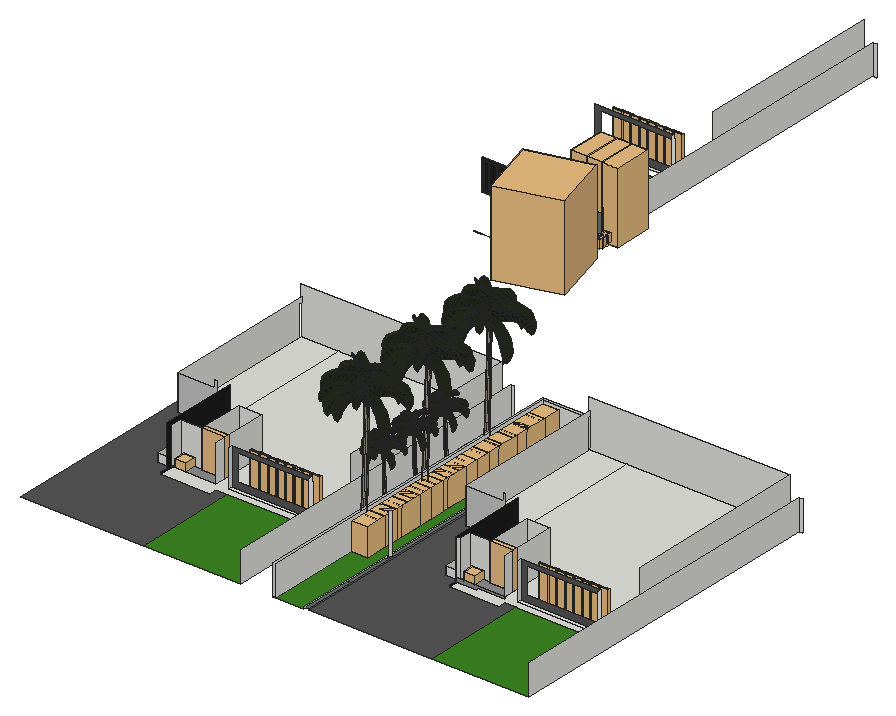
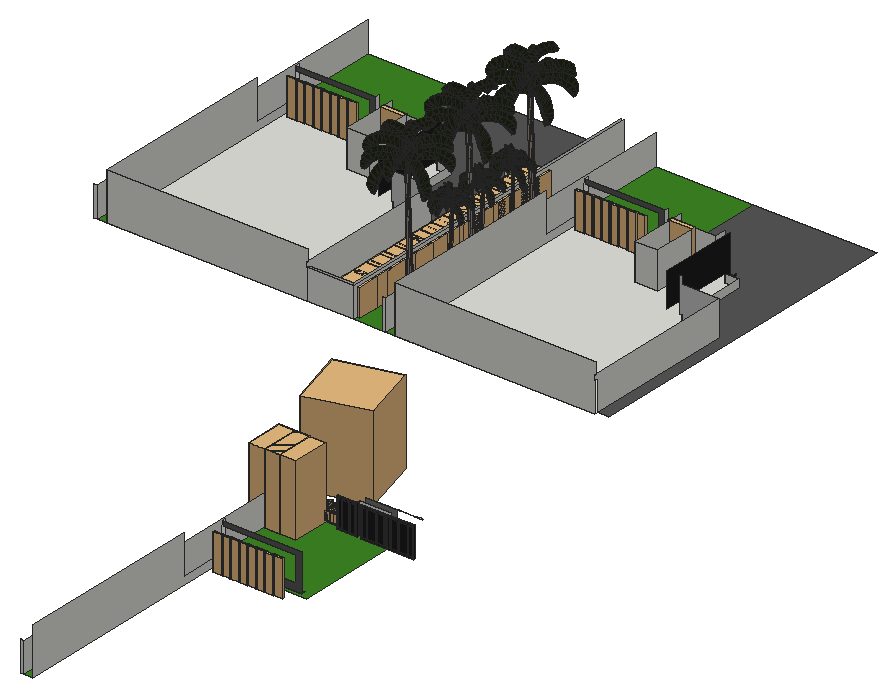
# SketchUp Ruby script. Lengths in inches.
U = 1.inch
M = Sketchup.active_model
def pt(a) = Geom::Point3d.new(a.map { |v| v * U })
def face(e, loops, mat)
  f = e.add_face(loops[0].map { |a| pt(a) })
  loops[1..].each { |l| e.add_face(l.map { |a| pt(a) }).erase! }
  f.material = f.back_material = mat if mat
  f
end
# faces: each face lists its corners as indices into pts; further lists are holes
def faces(e, pts, list, mat = nil) = list.each { |f| face(e, (f[0].is_a?(Array) ? f : [f]).map { |l| l.map { |i| pts[i] } }, mat) }
# xy, xz, yz: faces in a plane at the given z, y or x. An outline is a flat list of corners, or four numbers for a rectangle; further outlines are holes
def ring(l) = l.size == 4 ? [[l[0], l[1]], [l[2], l[1]], [l[2], l[3]], [l[0], l[3]]] : l.each_slice(2).to_a
def flat(e, list, mat, &to3) = list.each { |f| face(e, (f[0].is_a?(Array) ? f : [f]).map { |l| ring(l).map { |u, v| to3.(u, v) } }, mat) }
def xy(e, z, list, mat = nil) = flat(e, list, mat) { |x, y| [x, y, z] }
def xz(e, y, list, mat = nil) = flat(e, list, mat) { |x, z| [x, y, z] }
def yz(e, x, list, mat = nil) = flat(e, list, mat) { |y, z| [x, y, z] }
def lines(e, pts, list) = list.each { |a, b| e.add_line(pt(pts[a]), pt(pts[b])) }
# prism: a flat outline (further loops are holes) pulled along v
def prism(e, loops, v, mat = nil)
  f = face(e, loops, mat); d = Geom::Vector3d.new(v.map { |x| x * U })
  f.pushpull(f.normal.samedirection?(d) ? d.length : -d.length)
end
def box(e, o, s, mat = nil) = prism(e, [[o, [o[0] + s[0], o[1], o[2]], [o[0] + s[0], o[1] + s[1], o[2]], [o[0], o[1] + s[1], o[2]]]], [0, 0, s[2]], mat)
def at(x, y, z, deg = 0) = Geom::Transformation.translation(pt([x, y, z])) * Geom::Transformation.rotation(ORIGIN, Z_AXIS, deg.degrees)
def axes(o, x, y, z) = Geom::Transformation.new([*x, 0, *y, 0, *z, 0, *pt(o).to_a, 1])
def part(name) = M.definitions.add(name)
# library, detail: a bought-in or finely detailed component or shape, given as its bounding box
def library(name, o, s) = part(name).tap { |d| box(d.entities, o, s) }
def detail(e, o, s) = box(e.add_group.entities, o, s)
def put(e, d, t, mat = nil) = e.add_instance(d, t).tap { |i| i.material = mat if mat }
def group(e, t, mat = nil) = e.add_group.tap { |g| g.transformation = t; g.material = mat if mat }.entities
root = M.entities
M.materials.add("Antracyt").color = [44, 47, 50]
M.materials.add("Carpet_Ltblue").color = [157, 173, 165]
M.materials.add("Manila2").color = [36, 43, 22]
M.materials.add("ManilaTruck").color = [158, 143, 128]
M.materials.add("[Color M00]").color = [255, 255, 255]
M.materials.add("[Color M02]").color = [198, 198, 198]
M.materials.add("[Color M04]").color = [60, 133, 34]
M.materials.add("[Color M04]1").color = [142, 142, 142]
M.materials.add("[Color M05]1").color = [114, 114, 114]
M.materials.add("[Color M06]1").color = [86, 86, 86]
M.materials.add("[Color M08]").color = [30, 30, 30]
M.materials.add("[Color_F16]").color = [51, 102, 0]
M.materials.add("[Field Square Tile]").color = [217, 201, 169]
M.materials.add("[Slate Light Tile]").color = [86, 86, 86]
M.materials.add("[Slate]").color = [102, 110, 108]
c1 = part("Group\#102")
g1 = group(c1.entities,at(0,0,0))
prism(g1,[[[0,3,72],[70.5,3,72],[70.5,3,0],[0,3,0]],[[67.5,3,3],[67.5,3,69],[3,3,69],[3,3,3]]],[0,-3,0])
c2 = part("Group\#135")
box(c2.entities,[0,0,0],[0.5,1,66])
c3 = part("Group\#148")
box(c3.entities,[0,-1,0],[5.5,1,66])
box(c3.entities,[50.84,-1,0],[13.66,1,66])
box(c3.entities,[28.06,-1,0],[22.28,1,66])
box(c3.entities,[24.66,-1,0],[2.9,1,66])
box(c3.entities,[6,-1,0],[18.16,1,66])
c4 = part("Component\#23")
g2 = group(c4.entities,at(70.5,0,0),"[Color M08]")
put(g2,c1,axes([70.5,0,0],[-1,0,0],[0,1,0],[0,0,1]))
g3 = group(g2,at(3,2,3))
g4 = group(g3,at(0,-1,0))
box(g4,[0,0,0],[5.5,1,66])
box(g4,[50.84,0,0],[13.66,1,66])
box(g4,[28.06,0,0],[22.28,1,66])
box(g4,[24.66,0,0],[2.9,1,66])
box(g4,[6,0,0],[18.16,1,66])
put(g3,c2,axes([50.34,0,0],[1,0,0],[0,-1,0],[0,0,1]))
put(g3,c2,axes([24.16,0,0],[1,0,0],[0,-1,0],[0,0,1]))
put(g3,c2,axes([27.56,0,0],[1,0,0],[0,-1,0],[0,0,1]))
put(g3,c2,axes([5.5,0,0],[1,0,0],[0,-1,0],[0,0,1]))
g5 = group(c4.entities,at(70.5,0,0),"[Color M08]")
put(g5,c1,at(-70.5,0,0))
g6 = group(g5,at(-3,2,3,-180))
put(g6,c3,at(0,1,0))
put(g6,c2,at(50.34,0,0))
put(g6,c2,at(24.16,0,0))
put(g6,c2,at(27.56,0,0))
put(g6,c2,at(5.5,0,0))
g7 = group(c4.entities,at(150,0,0),"[Color M08]")
put(g7,c1,axes([54,0,0],[-0.76596,0,0],[0,1,0],[0,0,1]))
g8 = group(g7,at(2.3,2,3))
put(g8,c3,axes([0,-1,0],[0.76596,0,0],[0,-1,0],[0,0,1]))
put(g8,c2,axes([38.55,0,0],[0.76596,0,0],[0,-1,0],[0,0,1]))
put(g8,c2,axes([18.5,0,0],[0.76596,0,0],[0,-1,0],[0,0,1]))
put(g8,c2,axes([21.11,0,0],[0.76596,0,0],[0,-1,0],[0,0,1]))
put(g8,c2,axes([4.22,0,0],[0.76596,0,0],[0,-1,0],[0,0,1]))
c5 = library("Group\#1",[0,0,0],[29.75,5.78,110.95])
c6 = library("Obj_000004",[-25.54,-25.36,-14.31],[50.67,50.64,41.42])
c7 = library("Obj_000003",[-31,-31.06,-7.89],[62,62.12,39.58])
c8 = library("建立群組\#17",[-3.75,-3.74,-0.43],[25.39,25.39,17.69])
c9 = library("Potted plant",[-29.7,0,-10.87],[31.67,38.52,72.45])
c10 = library("Palm tree",[-4.09,-4.52,0],[193.52,193.51,258.93])
c11 = part("Palm+Tree")
put(c11.entities,c10,at(25.51,-21.81,0,15))
c12 = library("modern+door",[0,0,0],[59.06,11.8125,86.61])
c13 = part("P_trunck")
xz(c13.entities,2.71,[[7.39,73.15,8.49,73.15,9.26,91.63,8.16,91.63]],"ManilaTruck")
xz(c13.entities,6.09,[[3.91,10.2,7.39,73.15,8.49,73.15,5.33,10.2],[7.39,73.15,8.16,91.63,9.26,91.63,8.49,73.15]],"ManilaTruck")
p = [[3.19,0,0],[3.91,1.7,10.2],[2.75,2.54,10.2],[0.88,1.68,0],[6.05,0,0],[5.33,1.7,10.2],
  [8.36,1.68,0],[6.49,2.54,10.2],[2.31,3.9,10.2],[0,4.39,0],[9.24,4.39,0],[6.93,3.9,10.2],
  [2.75,5.25,10.2],[0.88,7.11,0],[8.36,7.11,0],[6.49,5.25,10.2],[3.91,6.09,10.2],[3.19,8.79,0],
  [6.05,8.79,0],[5.33,6.09,10.2],[7.39,2.71,73.15],[6.5,3.36,73.15],[8.49,2.71,73.15],[9.38,3.36,73.15],
  [6.16,4.4,73.15],[9.72,4.4,73.15],[6.5,5.45,73.15],[9.38,5.45,73.15],[7.39,6.09,73.15],[8.49,6.09,73.15],
  [8.16,2.71,91.63],[7.27,3.36,91.63],[10.15,3.36,91.63],[9.26,2.71,91.63],[6.93,4.4,91.63],[10.49,4.4,91.63],
  [7.27,5.45,91.63],[10.15,5.45,91.63],[8.16,6.09,91.63],[9.26,6.09,91.63]]
faces(c13.entities,p,[[0,1,2,3],[4,5,1,0],[6,7,5,4],[3,2,8,9],[6,10,11,7],[8,12,13,9],[11,10,14,15],[13,12,16,17],
  [18,19,15,14],[17,16,19,18],[1,20,21,2],[5,22,20,1],[7,23,22,5],[2,21,24,8],[7,11,25,23],[8,24,26,12],
  [11,15,27,25],[12,26,28,16],[19,29,27,15],[20,30,31,21],[23,32,33,22],[31,34,24,21],[23,25,35,32],[34,36,26,24],
  [25,27,37,35],[26,36,38,28],[29,39,37,27]],"ManilaTruck")
c14 = part("halfleave")
p = [[3.15,0,0],[0.57,2.5,1.86],[4.875,1.71,0],[46.16,1.62,0],[42.0625,6.98,0],[45.79,16.25,3.85],
  [48.16,12.12,1.98],[48.16,1.62,0],[6.6,3.42,0],[-0.25,5.68,3.48],[9.02,6.6,0],[-0.31,11.68,4.96],
  [2.05,16.625,5.9],[10.99,8.52,0],[36.71,10.67,0],[41.5,21.18,5.01],[8.2,21.17,6.52],[12.96,10.44,0],
  [15.16,24.88,6.8125],[17.61,12.89,0],[31.19,13.02,0],[36.16,23.66,5.26],[19.91,24.88,6.5625],[20.53,13.55,0],
  [25.77,13.9375,0],[30.57,24.88,6.0625],[25.21,24.88,6.26]]
faces(c14.entities,p,[[0,1,2],[3,4,5],[5,6,3],[7,3,6],[2,1,8],[9,8,1],[8,9,10],[11,10,9],
  [11,12,10],[13,10,12],[4,14,15],[15,5,4],[12,16,13],[17,13,16],[16,18,17],[19,17,18],
  [14,20,21],[21,15,14],[18,22,19],[23,19,22],[20,24,25],[25,21,20],[22,26,23],[24,23,26],
  [26,25,24]],"Manila2")
c15 = part("palmfronmanila")
put(c15.entities,c14,axes([0,0,4.06],[1,0,0],[0,1,0],[0,0,-1]))
put(c15.entities,c14,at(0,0,4.06))
c16 = part("manilafronnew")
put(c16.entities,c15,axes([0,16.76,11.56],[1,0,0],[0,0,1],[0,-1,0]))
c17 = part("Palm tree \#1")
put(c17.entities,c13,axes([-10.55,-3.84,0],[1.24992,0,0],[0,1.28016,0],[0,0,1.424]))
g9 = group(c17.entities,at(-43.54,-39.32,114.59))
put(g9,c16,axes([4.6,65.71,26.23],[0.53953,-0.65683,-0.22776],[0.61942,0.58508,-0.22],[0.31564,-0.02543,0.82105]))
put(g9,c16,axes([82.14,44.18,-7.44],[-0.84198,0.16366,0.22983],[-0.16944,-0.87168,0],[0.22561,-0.04385,0.85774]))
put(g9,c16,axes([74.79,11.41,2.76],[-0.448,0.77596,0],[-0.77596,-0.448,0],[0,0,0.896]))
put(g9,c16,axes([70.64,6.04,20.22],[-0.30809,0.82895,-0.08038],[-0.79676,-0.31832,-0.22889],[-0.24248,-0.00729,0.85422]))
put(g9,c16,axes([56.04,79.09,38.5],[-0.31814,-0.55104,-0.36736],[0.63629,-0.36736,0],[-0.18368,-0.31814,0.63629]))
put(g9,c16,axes([8.39,50.1,50.01],[0.44591,-0.25744,-0.51489],[0.36408,0.63061,0],[0.44591,-0.25744,0.51489]))
put(g9,c16,axes([8.53,12.03,22.52],[0.79394,0.3635,-0.23397],[-0.37632,0.82195,0],[0.21274,0.0974,0.8732]))
put(g9,c16,axes([54.07,81.55,-7.16],[-0.44094,-0.76373,0.19874],[0.78289,-0.452,0],[0.09937,0.17211,0.88188]))
put(g9,c16,axes([11.98,71.79,5.35],[0.444,-0.76903,0],[0.76903,0.444,0],[0,0,0.888]))
put(g9,c16,axes([-0.47,46.08,5.17],[0.83758,-0.34011,0],[0.34011,0.83758,0],[0,0,0.904]))
put(g9,c16,axes([35.85,3.71,-10.8],[0.42686,0.73934,0.2973],[-0.78289,0.452,0],[-0.14865,-0.25747,0.85372]))
put(g9,c16,axes([0.28,29.91,5.17],[0.904,0,0],[0,0.904,0],[0,0,0.904]))
put(g9,c16,axes([82.45,61.59,11.57],[-0.88287,-0.17622,-0.08182],[0.17259,-0.88617,0.04625],[-0.08923,0.02954,0.8991]))
put(g9,c16,axes([59.47,9.58,46.3125],[-0.10851,0.51281,-0.52416],[-0.72522,-0.15346,0],[-0.10851,0.51281,0.52416]))
c18 = part("עצי+דקל")
put(c18.entities,c17,axes([111.95,22.91,0],[1.33,0,0],[0,1.33,0],[0,0,1.33]))
put(c18.entities,c17,axes([230.0625,22.91,0],[1.33,0,0],[0,1.33,0],[0,0,1.33]))
put(c18.entities,c17,axes([348.17,22.91,0],[1.33,0,0],[0,1.33,0],[0,0,1.33]))
c19 = library("plant (1)",[-35.72,-28.42,0],[66.31,67.39,84.38])
xy(root,-19.75,[[1938.63,164.82,1946.07,164.82,1946.07,1192.15,2082.95,1192.15,2082.95,1201.875,1938.63,1201.875],[1354.48,464.0625,1504.89,464.0625,1504.89,487.3125,1810.23,487.3125,1810.23,1201.875,1310.86,1201.875,1310.86,505.3125,1354.48,505.3125],[2240.94,464.0625,2391.36,464.0625,2391.36,487.3125,2696.7,487.3125,2696.7,1201.875,2197.32,1201.875,2197.32,505.3125,2240.94,505.3125],[1196.48,726.125,1310.86,1201.875],[2082.95,726.125,2197.32,1201.875],
  [1208.96,1862.59,1214.07,1863.13,1219.05,1864.38,1196.62,1864.38,1198.77,1863.68,1203.82,1862.78],[1268.6,1864.08,1273.82,1864.38,1262.12,1864.38,1263.38,1864.23]])
xy(root,-19.75,[[1539.55,164.82,1838.4,164.82,1838.4,1201.875,1810.23,1201.875,1810.23,487.3125,1539.55,487.3125],[1946.07,164.82,2033.69,1192.15],[2426.02,164.82,2724.86,164.82,2724.86,1201.875,2696.7,1201.875,2696.7,487.3125,2426.02,487.3125],[1841.83,505.3125,1938.63,1201.875],[1474.1,1864.38,1481.1875,1995.38],
  [1171.82,2016.82,1470.67,2016.82,1470.67,3053.87,1442.5,3053.87,1442.5,2339.31,1171.82,2339.31]],"[Color M04]")
xy(root,-19.75,[[1161.04,164.82,1539.55,164.82,1539.55,487.3125,1504.89,487.3125,1504.89,464.0625,1354.48,464.0625,1354.48,505.3125,1310.86,505.3125,1310.86,726.125,1196.48,726.125,1196.48,1192.15,1161.04,1192.15],[2047.51,164.82,2426.02,164.82,2426.02,487.3125,2391.36,487.3125,2391.36,464.0625,2240.94,464.0625,2240.94,505.3125,2197.32,505.3125,2197.32,726.125,2082.95,726.125,2082.95,1192.15,2047.51,1192.15]],"[Slate Light Tile]")
xy(root,-19.3125,[[1474.1,1851.99,1481.1875,1864.38]],"[Field Square Tile]")
xy(root,-15.625,[[[2033.69,164.82,2047.51,1192.15],[2037.07,475.3125,2043.8,487.3125],[2037.07,322.71,2043.8,334.4375]]],"[Slate]")
xy(root,-3.75,[[1544.68,487.3125,1790.45,498.6875],[2431.15,487.3125,2676.91,498.6875],[1176.95,2339.31,1422.71,2350.68]])
xy(root,-2.375,[[1369.77,487.3125,1504.89,487.3125,1504.89,662.5,1434.68,662.5,1434.68,521.5625,1369.77,521.5625],[2256.23,487.3125,2391.36,487.3125,2391.36,662.5,2321.14,662.5,2321.14,521.5625,2256.23,521.5625]],"[Color M04]1")
xz(root,487.3125,[[2037.07,-15.625,2043.8,110.1875],[2240.94,-2.375,2256.23,110.1875]])
xz(root,487.3125,[[2240.94,-14.01,2306.98,-14.01,2306.98,-8.01,2391.36,-8.01,2391.36,-2.375,2240.94,-2.375]],"[Color M04]1")
xz(root,498.6875,[[1544.68,-3.75,1790.45,-3.75,1790.45,18.41,1563.99,18.41,1563.99,97.03,1790.45,97.03,1790.45,110.1875,1544.68,110.1875],[2431.15,-3.75,2676.91,-3.75,2676.91,18.41,2450.46,18.41,2450.46,97.03,2676.91,97.03,2676.91,110.1875,2431.15,110.1875]],"[Color M06]1")
xz(root,505.3125,[[1310.86,-19.75,1354.48,5.0625],[2197.32,-19.75,2240.94,5.0625]])
xz(root,521.5625,[[1369.77,-2.375,1434.68,110.1875],[2256.23,-2.375,2321.14,110.1875]])
xz(root,662.5,[[1434.68,-2.375,1504.89,110.1875],[2321.14,-2.375,2391.36,110.1875]])
xz(root,726.125,[[1196.48,-19.75,1310.86,-19.75,1310.86,5.0625,1316.04,5.0625,1316.04,110.1875,1310.86,110.1875,1310.86,88,1196.48,88],[2082.95,-19.75,2197.32,-19.75,2197.32,5.0625,2202.51,5.0625,2202.51,110.1875,2197.32,110.1875,2197.32,88,2082.95,88]],"[Color M02]")
xz(root,1192.15,[[1946.07,-19.75,2033.69,-19.75,2033.69,-15.625,2047.51,-15.625,2047.51,-19.75,2082.95,-19.75,2082.95,73,1946.07,73],[2033.69,-19.75,2047.51,-15.625]])
xz(root,1201.875,[[1196.48,-19.75,1196.48,88,1192.67,88,1192.67,125.0625,1810.23,125.0625,1810.23,-19.75],[1838.4,-19.75,1848.92,73],[1938.63,-19.75,2082.95,73],[2082.95,-19.75,2082.95,88,2079.13,88,2079.13,125.0625,2696.7,125.0625,2696.7,-19.75],[2724.86,-19.75,2735.38,73]])
xz(root,1864.38,[[1474.1,-19.75,1481.1875,-19.3125]])
xz(root,1995.38,[[1171.82,-19.75,1481.1875,-19.75,1481.1875,73,1419.92,73,1419.92,9.9375,1266.28,9.9375,1266.28,73,1171.82,73]],"[Color M05]1")
xz(root,2016.82,[[1171.82,-19.75,1266.28,73],[1266.28,-19.75,1419.92,9.9375],[1419.92,-19.75,1470.67,73]])
xz(root,2350.68,[[1176.95,-3.75,1422.71,-3.75,1422.71,18.41,1196.26,18.41,1196.26,97.03,1422.71,97.03,1422.71,110.1875,1176.95,110.1875]],"[Color M06]1")
xz(root,3053.87,[[1470.67,-19.75,1481.1875,73]])
yz(root,1196.48,[[726.125,-19.75,726.125,88,1201.875,88,1201.875,73,1192.15,73,1192.15,-19.75]])
yz(root,1310.86,[[505.3125,-19.75,726.125,5.0625]])
yz(root,1354.48,[[464.0625,-19.75,464.0625,-14.01,487.3125,-14.01,487.3125,110.1875,726.125,110.1875,726.125,5.0625,505.3125,5.0625,505.3125,-19.75]],"[Color M08]")
yz(root,1369.77,[[487.3125,-2.375,521.5625,110.1875]])
yz(root,1422.71,[[2339.31,-3.75,2339.31,110.1875,2350.68,110.1875,2350.68,97.03,2353.71,97.03,2353.71,18.41,2350.68,18.41,2350.68,-3.75]],"[Color M00]")
yz(root,1434.68,[[521.5625,-2.375,662.5,110.1875]])
yz(root,1442.5,[[2339.31,-19.75,3053.87,-19.75,3053.87,125.0625,2475.84,125.0625,2475.84,5.0625,2339.31,5.0625]])
yz(root,1470.67,[[2016.82,-19.75,3053.87,73]])
yz(root,1504.89,[[487.3125,-2.375,662.5,110.1875]])
yz(root,1544.68,[[487.3125,-3.75,498.6875,110.1875]])
yz(root,1790.45,[[487.3125,-3.75,487.3125,110.1875,498.6875,110.1875,498.6875,97.03,501.72,97.03,501.72,18.41,498.6875,18.41,498.6875,-3.75]],"[Color M00]")
yz(root,1810.23,[[487.3125,-19.75,1201.875,-19.75,1201.875,125.0625,623.84,125.0625,623.84,5.0625,487.3125,5.0625]])
yz(root,1838.4,[[164.82,-19.75,1201.875,73]])
yz(root,1938.63,[[164.82,-19.75,1201.875,73]])
yz(root,1946.07,[[164.82,-19.75,1192.15,73]])
yz(root,2033.69,[[164.82,-19.75,1192.15,-15.625]])
yz(root,2047.51,[[164.82,-19.75,1192.15,-15.625]],"[Slate]")
yz(root,2082.95,[[726.125,-19.75,726.125,88,1201.875,88,1201.875,73,1192.15,73,1192.15,-19.75]])
yz(root,2197.32,[[505.3125,-19.75,726.125,5.0625]])
yz(root,2240.94,[[464.0625,-19.75,464.0625,-14.01,487.3125,-14.01,487.3125,110.1875,726.125,110.1875,726.125,5.0625,505.3125,5.0625,505.3125,-19.75]],"[Color M08]")
yz(root,2256.23,[[487.3125,-2.375,521.5625,110.1875]])
yz(root,2321.14,[[521.5625,-2.375,662.5,110.1875]])
yz(root,2391.36,[[487.3125,-2.375,662.5,110.1875]])
yz(root,2431.15,[[487.3125,-3.75,498.6875,110.1875]])
yz(root,2676.91,[[487.3125,-3.75,487.3125,110.1875,498.6875,110.1875,498.6875,97.03,501.72,97.03,501.72,18.41,498.6875,18.41,498.6875,-3.75]],"[Color M00]")
yz(root,2696.7,[[487.3125,-19.75,1201.875,-19.75,1201.875,125.0625,623.84,125.0625,623.84,5.0625,487.3125,5.0625]])
yz(root,2724.86,[[164.82,-19.75,1201.875,73]])
p = [[1219.05,1864.38,-19.75],[1262.12,1864.38,-19.75],[1219.05,1864.38,-19.3125],[1474.1,1864.38,-19.3125],[1273.82,1864.38,-19.75],[1474.1,1864.38,-19.75]]
lines(root,p,[[0,1],[2,3],[4,5]])
put(root,c4,axes([1090.68,2027.05,-19.75],[1.16,0,0],[0,1.16,0],[0,0,1.28819]))
put(root,c5,at(1209.28,2379.4,-13.92),"[Color M04]")
put(root,c6,axes([1230.62,1982.25,-8.96],[0.64,0,0],[0,0.64,0],[0,0,0.64]))
put(root,c6,axes([1246.49,1982.25,-8.96],[0.64,0,0],[0,0.64,0],[0,0,0.64]))
put(root,c7,axes([1246.49,1982.25,-8.96],[0.64,0,0],[0,0.64,0],[0,0,0.64]),"[Color_F16]")
put(root,c6,axes([1246.9,1982.18,-8.96],[0.45255,0.45255,-0.00035],[-0.45255,0.45255,0.00015],[0.00035,0.00015,0.64]))
put(root,c7,axes([1246.9,1982.18,-8.96],[0.45255,0.45255,-0.00035],[-0.45255,0.45255,0.00015],[0.00035,0.00015,0.64]),"[Color_F16]")
put(root,c5,at(1235.68,2380.96,-13.92),"[Color M04]")
put(root,c7,axes([1262.73,1983.12,-8.96],[-0.54627,0.33345,-0.00035],[-0.33345,-0.54627,0.00015],[-0.00023,0.00031,0.64]),"[Color_F16]")
put(root,c7,axes([1262.75,1982.71,-8.96],[-0.15049,0.62206,0],[-0.62206,-0.15049,0],[0,0,0.64]),"[Color_F16]")
put(root,c6,axes([1262.75,1982.71,-8.96],[-0.15049,0.62206,0],[-0.62206,-0.15049,0],[0,0,0.64]))
put(root,c6,axes([1262.73,1983.12,-8.96],[-0.54627,0.33345,-0.00035],[-0.33345,-0.54627,0.00015],[-0.00023,0.00031,0.64]))
put(root,c5,at(1262.65,2380.96,-13.92),"[Color M04]")
put(root,c6,axes([1278.24,1982.25,-8.96],[0.64,0,0],[0,0.64,0],[0,0,0.64]))
put(root,c7,axes([1278.24,1982.25,-8.96],[0.64,0,0],[0,0.64,0],[0,0,0.64]),"[Color_F16]")
put(root,c6,axes([1278.65,1982.18,-8.96],[0.45255,0.45255,-0.00035],[-0.45255,0.45255,0.00015],[0.00035,0.00015,0.64]))
put(root,c7,axes([1278.65,1982.18,-8.96],[0.45255,0.45255,-0.00035],[-0.45255,0.45255,0.00015],[0.00035,0.00015,0.64]),"[Color_F16]")
put(root,c6,axes([1294.12,1982.25,-8.96],[0.64,0,0],[0,0.64,0],[0,0,0.64]))
put(root,c7,axes([1294.12,1982.25,-8.96],[0.64,0,0],[0,0.64,0],[0,0,0.64]),"[Color_F16]")
put(root,c6,axes([1294.53,1982.18,-8.96],[0.45255,0.45255,-0.00035],[-0.45255,0.45255,0.00015],[0.00035,0.00015,0.64]))
put(root,c7,axes([1294.53,1982.18,-8.96],[0.45255,0.45255,-0.00035],[-0.45255,0.45255,0.00015],[0.00035,0.00015,0.64]),"[Color_F16]")
put(root,c5,at(1288.71,2380.96,-13.92),"[Color M04]")
put(root,c6,axes([1309.7,1982.52,-8.96],[0.28256,0.57425,0],[-0.57425,0.28256,0],[0,0,0.64]))
put(root,c7,axes([1309.95,1982.85,-8.96],[-0.20625,0.60586,-0.00035],[-0.60586,-0.20625,0.00015],[0.00002,0.00038,0.64]),"[Color_F16]")
put(root,c7,axes([1309.99,1982.25,-8.96],[0.64,0,0],[0,0.64,0],[0,0,0.64]),"[Color_F16]")
put(root,c6,axes([1309.95,1982.85,-8.96],[-0.20625,0.60586,-0.00035],[-0.60586,-0.20625,0.00015],[0.00002,0.00038,0.64]))
put(root,c6,axes([1324.46,1996.2,-8.16],[0.64,0,0],[0,0.64,0],[0,0,0.64]))
put(root,c5,at(1314.78,2380.96,-13.92),"[Color M04]")
put(root,c6,axes([1340.33,1996.2,-8.16],[0.64,0,0],[0,0.64,0],[0,0,0.64]))
put(root,c7,axes([1340.33,1996.2,-8.16],[0.64,0,0],[0,0.64,0],[0,0,0.64]),"[Color_F16]")
put(root,c6,axes([1340.74,1996.125,-8.16],[0.45255,0.45255,-0.00035],[-0.45255,0.45255,0.00015],[0.00035,0.00015,0.64]))
put(root,c7,axes([1340.74,1996.125,-8.16],[0.45255,0.45255,-0.00035],[-0.45255,0.45255,0.00015],[0.00035,0.00015,0.64]),"[Color_F16]")
put(root,c5,at(1340.84,2380.96,-13.92),"[Color M04]")
put(root,c7,axes([1356.57,1997.07,-8.16],[-0.54627,0.33345,-0.00035],[-0.33345,-0.54627,0.00015],[-0.00023,0.00031,0.64]),"[Color_F16]")
put(root,c7,axes([1356.59,1996.66,-8.16],[-0.15049,0.62206,0],[-0.62206,-0.15049,0],[0,0,0.64]),"[Color_F16]")
put(root,c6,axes([1356.59,1996.66,-8.16],[-0.15049,0.62206,0],[-0.62206,-0.15049,0],[0,0,0.64]))
put(root,c6,axes([1356.57,1997.07,-8.16],[-0.54627,0.33345,-0.00035],[-0.33345,-0.54627,0.00015],[-0.00023,0.00031,0.64]))
put(root,c6,axes([1372.08,1996.2,-8.16],[0.64,0,0],[0,0.64,0],[0,0,0.64]))
put(root,c7,axes([1372.08,1996.2,-8.16],[0.64,0,0],[0,0.64,0],[0,0,0.64]),"[Color_F16]")
put(root,c6,axes([1372.49,1996.125,-8.16],[0.45255,0.45255,-0.00035],[-0.45255,0.45255,0.00015],[0.00035,0.00015,0.64]))
put(root,c7,axes([1372.49,1996.125,-8.16],[0.45255,0.45255,-0.00035],[-0.45255,0.45255,0.00015],[0.00035,0.00015,0.64]),"[Color_F16]")
put(root,c5,at(1366.9,2380.96,-13.92),"[Color M04]")
put(root,c6,axes([1387.95,1996.2,-8.16],[0.64,0,0],[0,0.64,0],[0,0,0.64]))
put(root,c7,axes([1387.95,1996.2,-8.16],[0.64,0,0],[0,0.64,0],[0,0,0.64]),"[Color_F16]")
put(root,c6,axes([1388.36,1996.125,-8.16],[0.45255,0.45255,-0.00035],[-0.45255,0.45255,0.00015],[0.00035,0.00015,0.64]))
put(root,c7,axes([1388.36,1996.125,-8.16],[0.45255,0.45255,-0.00035],[-0.45255,0.45255,0.00015],[0.00035,0.00015,0.64]),"[Color_F16]")
put(root,c6,axes([1394.83,1996.2,-8.16],[0.64,0,0],[0,0.64,0],[0,0,0.64]))
put(root,c8,axes([1383.75,492.33,-1.8],[1.341,0,0],[0,1.341,0],[0,0,1.341]),"Carpet_Ltblue")
put(root,c6,axes([1403.54,1996.47,-8.16],[0.28256,0.57425,0],[-0.57425,0.28256,0],[0,0,0.64]))
put(root,c7,axes([1403.79,1996.8,-8.16],[-0.20625,0.60586,-0.00035],[-0.60586,-0.20625,0.00015],[0.00002,0.00038,0.64]),"[Color_F16]")
put(root,c7,axes([1403.83,1996.2,-8.16],[0.64,0,0],[0,0.64,0],[0,0,0.64]),"[Color_F16]")
put(root,c6,axes([1403.79,1996.8,-8.16],[-0.20625,0.60586,-0.00035],[-0.60586,-0.20625,0.00015],[0.00002,0.00038,0.64]))
put(root,c5,at(1392.96,2380.96,-13.92),"[Color M04]")
put(root,c6,axes([1410.71,1996.2,-8.16],[0.64,0,0],[0,0.64,0],[0,0,0.64]))
put(root,c7,axes([1410.71,1996.2,-8.16],[0.64,0,0],[0,0.64,0],[0,0,0.64]),"[Color_F16]")
put(root,c6,axes([1411.12,1996.125,-8.16],[0.45255,0.45255,-0.00035],[-0.45255,0.45255,0.00015],[0.00035,0.00015,0.64]))
put(root,c7,axes([1411.12,1996.125,-8.16],[0.45255,0.45255,-0.00035],[-0.45255,0.45255,0.00015],[0.00035,0.00015,0.64]),"[Color_F16]")
put(root,c9,axes([1460.77,2016.82,12.86],[3,0,0],[0,3,0],[0,0,3]))
put(root,c7,axes([1426.94,1997.07,-8.16],[-0.54627,0.33345,-0.00035],[-0.33345,-0.54627,0.00015],[-0.00023,0.00031,0.64]),"[Color_F16]")
put(root,c7,axes([1426.96,1996.66,-8.16],[-0.15049,0.62206,0],[-0.62206,-0.15049,0],[0,0,0.64]),"[Color_F16]")
put(root,c6,axes([1426.96,1996.66,-8.16],[-0.15049,0.62206,0],[-0.62206,-0.15049,0],[0,0,0.64]))
put(root,c6,axes([1426.94,1997.07,-8.16],[-0.54627,0.33345,-0.00035],[-0.33345,-0.54627,0.00015],[-0.00023,0.00031,0.64]))
put(root,c6,axes([1442.45,1996.2,-8.16],[0.64,0,0],[0,0.64,0],[0,0,0.64]))
put(root,c7,axes([1442.45,1996.2,-8.16],[0.64,0,0],[0,0.64,0],[0,0,0.64]),"[Color_F16]")
put(root,c6,axes([1442.86,1996.125,-8.16],[0.45255,0.45255,-0.00035],[-0.45255,0.45255,0.00015],[0.00035,0.00015,0.64]))
put(root,c7,axes([1442.86,1996.125,-8.16],[0.45255,0.45255,-0.00035],[-0.45255,0.45255,0.00015],[0.00035,0.00015,0.64]),"[Color_F16]")
put(root,c11,at(1356.11,1726.87,-17.22))
put(root,c6,axes([1458.33,1996.2,-8.16],[0.64,0,0],[0,0.64,0],[0,0,0.64]))
put(root,c7,axes([1458.33,1996.2,-8.16],[0.64,0,0],[0,0.64,0],[0,0,0.64]),"[Color_F16]")
put(root,c6,axes([1458.74,1996.125,-8.16],[0.45255,0.45255,-0.00035],[-0.45255,0.45255,0.00015],[0.00035,0.00015,0.64]))
put(root,c7,axes([1458.74,1996.125,-8.16],[0.45255,0.45255,-0.00035],[-0.45255,0.45255,0.00015],[0.00035,0.00015,0.64]),"[Color_F16]")
put(root,c9,axes([1510.64,2016.82,12.86],[3,0,0],[0,3,0],[0,0,3]))
put(root,c12,axes([1434.68,519.08,-2.375],[1.21,0,0],[0,1.21,0],[0,0,1.32195]),"Antracyt")
put(root,c6,axes([1473.92,1996.47,-8.16],[0.28256,0.57425,0],[-0.57425,0.28256,0],[0,0,0.64]))
put(root,c7,axes([1474.17,1996.8,-8.16],[-0.20625,0.60586,-0.00035],[-0.60586,-0.20625,0.00015],[0.00002,0.00038,0.64]),"[Color_F16]")
put(root,c7,axes([1474.2,1996.2,-8.16],[0.64,0,0],[0,0.64,0],[0,0,0.64]),"[Color_F16]")
put(root,c6,axes([1474.17,1996.8,-8.16],[-0.20625,0.60586,-0.00035],[-0.60586,-0.20625,0.00015],[0.00002,0.00038,0.64]))
put(root,c5,at(1577.02,527.41,-13.92),"[Color M04]")
put(root,c5,at(1603.41,528.96,-13.92),"[Color M04]")
put(root,c5,at(1630.38,528.96,-13.92),"[Color M04]")
put(root,c5,at(1656.45,528.96,-13.92),"[Color M04]")
put(root,c5,at(1682.51,528.96,-13.92),"[Color M04]")
put(root,c5,at(1708.57,528.96,-13.92),"[Color M04]")
put(root,c5,at(1734.63,528.96,-13.92),"[Color M04]")
put(root,c5,at(1760.7,528.96,-13.92),"[Color M04]")
put(root,c18,at(1875.53,983.67,-19.75,-90))
put(root,c18,axes([1962.42,332.28,-19.75],[0,2,0],[-2,0,0],[0,0,2]))
put(root,c19,at(1966.18,482.67,-19.75))
put(root,c19,at(1966.18,526.98,-19.75))
put(root,c19,at(1966.18,571.3,-19.75))
put(root,c19,at(1966.18,615.61,-19.75))
put(root,c19,at(1966.18,659.92,-19.75))
put(root,c19,at(1966.18,704.23,-19.75))
put(root,c19,at(1966.18,748.55,-19.75))
put(root,c19,at(1966.18,792.86,-19.75))
put(root,c19,at(1966.18,837.17,-19.75))
put(root,c19,at(1966.18,881.48,-19.75))
put(root,c19,at(1966.18,935.3,-19.75))
put(root,c19,at(1966.18,989.11,-19.75))
put(root,c19,at(1966.18,1042.92,-19.75))
put(root,c19,at(1966.18,1096.73,-19.75))
put(root,c19,at(1966.18,1150.55,-19.75))
put(root,c8,axes([2270.21,492.33,-1.8],[1.341,0,0],[0,1.341,0],[0,0,1.341]),"Carpet_Ltblue")
put(root,c12,axes([2321.14,519.08,-2.375],[1.21,0,0],[0,1.21,0],[0,0,1.32195]),"Antracyt")
put(root,c5,at(2463.48,527.41,-13.92),"[Color M04]")
put(root,c5,at(2489.88,528.96,-13.92),"[Color M04]")
put(root,c5,at(2516.85,528.96,-13.92),"[Color M04]")
put(root,c5,at(2542.91,528.96,-13.92),"[Color M04]")
put(root,c5,at(2568.97,528.96,-13.92),"[Color M04]")
put(root,c5,at(2595.03,528.96,-13.92),"[Color M04]")
put(root,c5,at(2621.1,528.96,-13.92),"[Color M04]")
put(root,c5,at(2647.16,528.96,-13.92),"[Color M04]")
